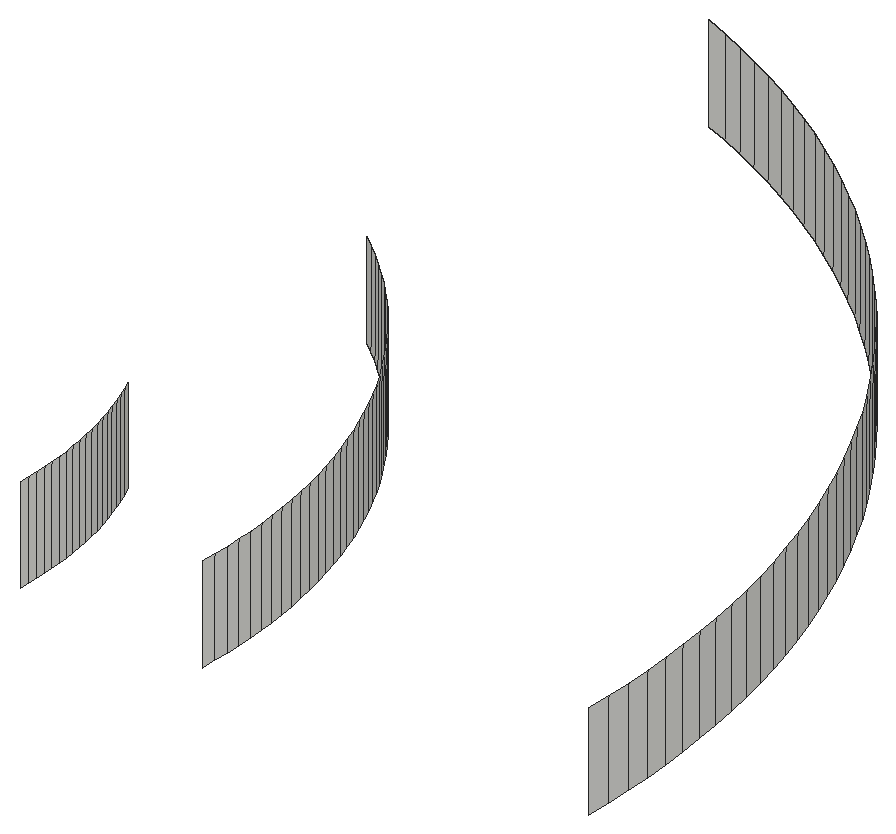
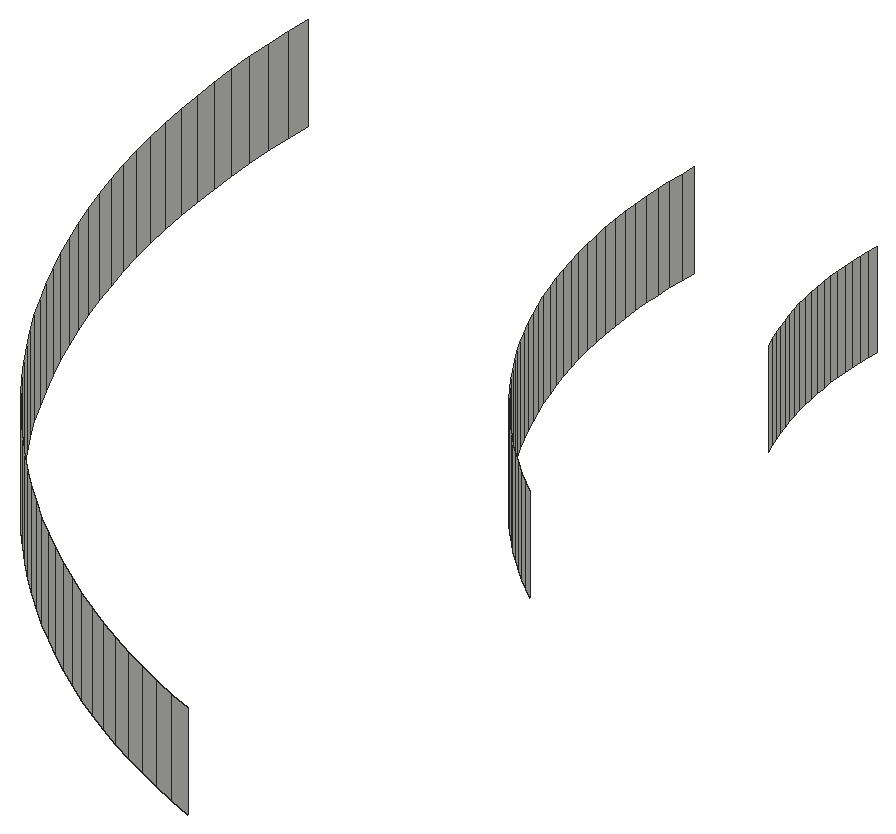
# SketchUp Ruby script. Lengths in inches.
U = 1.inch
M = Sketchup.active_model
def pt(a) = Geom::Point3d.new(a.map { |v| v * U })
def face(e, loops, mat)
  f = e.add_face(loops[0].map { |a| pt(a) })
  loops[1..].each { |l| e.add_face(l.map { |a| pt(a) }).erase! }
  f.material = f.back_material = mat if mat
  f
end
# faces: each face lists its corners as indices into pts; further lists are holes
def faces(e, pts, list, mat = nil) = list.each { |f| face(e, (f[0].is_a?(Array) ? f : [f]).map { |l| l.map { |i| pts[i] } }, mat) }
# xy, xz, yz: faces in a plane at the given z, y or x. An outline is a flat list of corners, or four numbers for a rectangle; further outlines are holes
def ring(l) = l.size == 4 ? [[l[0], l[1]], [l[2], l[1]], [l[2], l[3]], [l[0], l[3]]] : l.each_slice(2).to_a
def flat(e, list, mat, &to3) = list.each { |f| face(e, (f[0].is_a?(Array) ? f : [f]).map { |l| ring(l).map { |u, v| to3.(u, v) } }, mat) }
def xy(e, z, list, mat = nil) = flat(e, list, mat) { |x, y| [x, y, z] }
def xz(e, y, list, mat = nil) = flat(e, list, mat) { |x, z| [x, y, z] }
def yz(e, x, list, mat = nil) = flat(e, list, mat) { |y, z| [x, y, z] }
def lines(e, pts, list) = list.each { |a, b| e.add_line(pt(pts[a]), pt(pts[b])) }
# prism: a flat outline (further loops are holes) pulled along v
def prism(e, loops, v, mat = nil)
  f = face(e, loops, mat); d = Geom::Vector3d.new(v.map { |x| x * U })
  f.pushpull(f.normal.samedirection?(d) ? d.length : -d.length)
end
def box(e, o, s, mat = nil) = prism(e, [[o, [o[0] + s[0], o[1], o[2]], [o[0] + s[0], o[1] + s[1], o[2]], [o[0], o[1] + s[1], o[2]]]], [0, 0, s[2]], mat)
def at(x, y, z, deg = 0) = Geom::Transformation.translation(pt([x, y, z])) * Geom::Transformation.rotation(ORIGIN, Z_AXIS, deg.degrees)
def axes(o, x, y, z) = Geom::Transformation.new([*x, 0, *y, 0, *z, 0, *pt(o).to_a, 1])
def part(name) = M.definitions.add(name)
# library, detail: a bought-in or finely detailed component or shape, given as its bounding box
def library(name, o, s) = part(name).tap { |d| box(d.entities, o, s) }
def detail(e, o, s) = box(e.add_group.entities, o, s)
def put(e, d, t, mat = nil) = e.add_instance(d, t).tap { |i| i.material = mat if mat }
def group(e, t, mat = nil) = e.add_group.tap { |g| g.transformation = t; g.material = mat if mat }.entities
root = M.entities
p = [[941.97,324.3125,117.3125],[941.93,323.37,117.3125],[941.93,323.37,111.3125],[941.97,324.3125,111.3125],[965.96,323.6875,117.3125],[965.98,325.26,117.3125],
  [965.98,325.26,111.3125],[965.96,323.6875,111.3125],[929.95,324,117.3125],[929.97,324.63,117.3125],[929.97,324.63,111.3125],[929.95,324,111.3125],
  [941.98,325.26,117.3125],[941.98,325.26,111.3125],[929.98,325.26,117.3125],[929.98,325.26,111.3125],[929.97,325.88,117.3125],[929.97,325.88,111.3125],
  [941.97,326.2,117.3125],[941.97,326.2,111.3125],[965.96,326.83,117.3125],[965.96,326.83,111.3125],[929.95,326.51,117.3125],[929.95,326.51,111.3125],
  [941.93,327.14,117.3125],[941.93,327.14,111.3125],[929.9,327.14,117.3125],[929.9,327.14,111.3125],[965.9,328.4,117.3125],[965.9,328.4,111.3125],
  [929.85,327.76,117.3125],[929.85,327.76,111.3125],[941.87,328.08,117.3125],[941.87,328.08,111.3125],[929.77,328.39,117.3125],[929.77,328.39,111.3125],
  [941.78,329.02,117.3125],[941.78,329.02,111.3125],[929.68,329.01,117.3125],[929.68,329.01,111.3125],[965.79,329.96,117.3125],[965.79,329.96,111.3125],
  [929.58,329.63,117.3125],[929.58,329.63,111.3125],[941.67,329.96,117.3125],[941.67,329.96,111.3125],[929.45,330.25,117.3125],[929.45,330.25,111.3125],
  [941.54,330.89,117.3125],[941.54,330.89,111.3125],[965.65,331.53,117.3125],[965.65,331.53,111.3125],[929.32,330.86,117.3125],[929.32,330.86,111.3125],
  [929.16,331.47,117.3125],[929.16,331.47,111.3125],[941.375,331.82,117.3125],[941.375,331.82,111.3125],[928.99,332.07,117.3125],[928.99,332.07,111.3125],
  [965.47,333.09,117.3125],[965.47,333.09,111.3125],[941.19,332.74,117.3125],[941.19,332.74,111.3125],[928.8,332.67,117.3125],[928.8,332.67,111.3125],
  [928.6,333.27,117.3125],[928.6,333.27,111.3125],[940.98,333.66,117.3125],[940.98,333.66,111.3125],[965.24,334.64,117.3125],[965.24,334.64,111.3125],
  [928.38,333.86,117.3125],[928.38,333.86,111.3125],[940.75,334.57,117.3125],[940.75,334.57,111.3125],[928.15,334.44,117.3125],[928.15,334.44,111.3125],
  [927.9,335.02,117.3125],[927.9,335.02,111.3125],[940.5,335.48,117.3125],[940.5,335.48,111.3125],[964.97,336.19,117.3125],[964.97,336.19,111.3125],
  [940.22,336.38,117.3125],[940.22,336.38,111.3125],[964.67,337.73,117.3125],[964.67,337.73,111.3125],[939.91,337.27,117.3125],[939.91,337.27,111.3125],
  [939.59,338.16,117.3125],[939.59,338.16,111.3125],[964.32,339.26,117.3125],[964.32,339.26,111.3125],[939.24,339.03,117.3125],[939.24,339.03,111.3125],
  [938.87,339.9,117.3125],[938.87,339.9,111.3125],[963.93,340.79,117.3125],[963.93,340.79,111.3125],[938.47,340.75,117.3125],[938.47,340.75,111.3125],
  [938.05,341.6,117.3125],[938.05,341.6,111.3125],[963.51,342.3,117.3125],[963.51,342.3,111.3125],[937.62,342.43,117.3125],[937.62,342.43,111.3125],
  [963.04,343.8,117.3125],[963.04,343.8,111.3125],[937.16,343.26,117.3125],[937.16,343.26,111.3125],[936.67,344.07,117.3125],[936.67,344.07,111.3125],
  [962.54,345.28,117.3125],[962.54,345.28,111.3125],[936.17,344.86,117.3125],[936.17,344.86,111.3125],[935.65,345.65,117.3125],[935.65,345.65,111.3125],
  [961.99,346.76,117.3125],[961.99,346.76,111.3125],[935.1,346.42,117.3125],[935.1,346.42,111.3125],[934.54,347.17,117.3125],[934.54,347.17,111.3125],
  [961.41,348.22,117.3125],[961.41,348.22,111.3125],[933.96,347.91,117.3125],[933.96,347.91,111.3125],[933.35,348.64,117.3125],[933.35,348.64,111.3125],
  [960.79,349.66,117.3125],[960.79,349.66,111.3125],[932.73,349.34,117.3125],[932.73,349.34,111.3125],[932.09,350.04,117.3125],[932.09,350.04,111.3125],
  [960.13,351.09,117.3125],[960.13,351.09,111.3125],[931.43,350.71,117.3125],[931.43,350.71,111.3125],[930.76,351.37,117.3125],[930.76,351.37,111.3125],
  [959.4375,352.5,117.3125],[959.4375,352.5,111.3125],[930.07,352.01,117.3125],[930.07,352.01,111.3125],[929.36,352.63,117.3125],[929.36,352.63,111.3125],
  [958.71,353.89,117.3125],[958.71,353.89,111.3125],[928.63,353.23,117.3125],[928.63,353.23,111.3125],[927.89,353.82,117.3125],[927.89,353.82,111.3125],
  [957.94,355.26,117.3125],[957.94,355.26,111.3125],[957.14,356.61,117.3125],[957.14,356.61,111.3125],[956.3,357.93,117.3125],[956.3,357.93,111.3125],
  [955.43,359.24,117.3125],[955.43,359.24,111.3125],[954.52,360.52,117.3125],[954.52,360.52,111.3125],[953.58,361.78,117.3125],[953.58,361.78,111.3125],
  [952.61,363.02,117.3125],[952.61,363.02,111.3125],[951.6,364.22,117.3125],[951.6,364.22,111.3125],[950.57,365.4,117.3125],[950.57,365.4,111.3125],
  [949.5,366.56,117.3125],[949.5,366.56,111.3125],[948.41,367.68,117.3125],[948.41,367.68,111.3125],[947.28,368.78,117.3125],[947.28,368.78,111.3125],
  [946.125,369.84,117.3125],[946.125,369.84,111.3125],[944.95,370.88,117.3125],[944.95,370.88,111.3125],[943.74,371.88,117.3125],[943.74,371.88,111.3125],
  [942.5,372.86,117.3125],[942.5,372.86,111.3125],[941.25,373.8,117.3125],[941.25,373.8,111.3125],[939.96,374.7,117.3125],[939.96,374.7,111.3125],
  [938.66,375.58,117.3125],[938.66,375.58,111.3125],[937.33,376.41,117.3125],[937.33,376.41,111.3125],[935.98,377.22,117.3125],[935.98,377.22,111.3125],
  [934.61,377.99,117.3125],[934.61,377.99,111.3125],[933.22,378.72,117.3125],[933.22,378.72,111.3125],[931.81,379.41,117.3125],[931.81,379.41,111.3125],
  [930.38,380.07,117.3125],[930.38,380.07,111.3125],[928.94,380.6875,117.3125],[928.94,380.6875,111.3125],[927.48,381.27,117.3125],[927.48,381.27,111.3125]]
faces(root,p,[[0,1,2,3],[4,5,6,7],[8,9,10,11],[12,0,3,13],[9,14,15,10],[14,16,17,15],[18,12,13,19],[5,20,21,6],
  [16,22,23,17],[24,18,19,25],[22,26,27,23],[20,28,29,21],[26,30,31,27],[32,24,25,33],[30,34,35,31],[36,32,33,37],
  [34,38,39,35],[28,40,41,29],[38,42,43,39],[44,36,37,45],[42,46,47,43],[48,44,45,49],[40,50,51,41],[46,52,53,47],
  [52,54,55,53],[56,48,49,57],[54,58,59,55],[50,60,61,51],[62,56,57,63],[58,64,65,59],[64,66,67,65],[68,62,63,69],
  [60,70,71,61],[66,72,73,67],[74,68,69,75],[72,76,77,73],[76,78,79,77],[80,74,75,81],[70,82,83,71],[84,80,81,85],
  [82,86,87,83],[88,84,85,89],[90,88,89,91],[86,92,93,87],[94,90,91,95],[96,94,95,97],[92,98,99,93],[100,96,97,101],
  [102,100,101,103],[98,104,105,99],[106,102,103,107],[104,108,109,105],[110,106,107,111],[112,110,111,113],[108,114,115,109],[116,112,113,117],
  [118,116,117,119],[114,120,121,115],[122,118,119,123],[124,122,123,125],[120,126,127,121],[128,124,125,129],[130,128,129,131],[126,132,133,127],
  [134,130,131,135],[136,134,135,137],[132,138,139,133],[140,136,137,141],[142,140,141,143],[138,144,145,139],[146,142,143,147],[148,146,147,149],
  [144,150,151,145],[152,148,149,153],[154,152,153,155],[150,156,157,151],[156,158,159,157],[158,160,161,159],[160,162,163,161],[162,164,165,163],
  [164,166,167,165],[166,168,169,167],[168,170,171,169],[170,172,173,171],[172,174,175,173],[174,176,177,175],[176,178,179,177],[178,180,181,179],
  [180,182,183,181],[182,184,185,183],[184,186,187,185],[186,188,189,187],[188,190,191,189],[190,192,193,191],[192,194,195,193],[194,196,197,195],
  [196,198,199,197],[198,200,201,199],[200,202,203,201],[202,204,205,203],[204,206,207,205],[206,208,209,207]])
